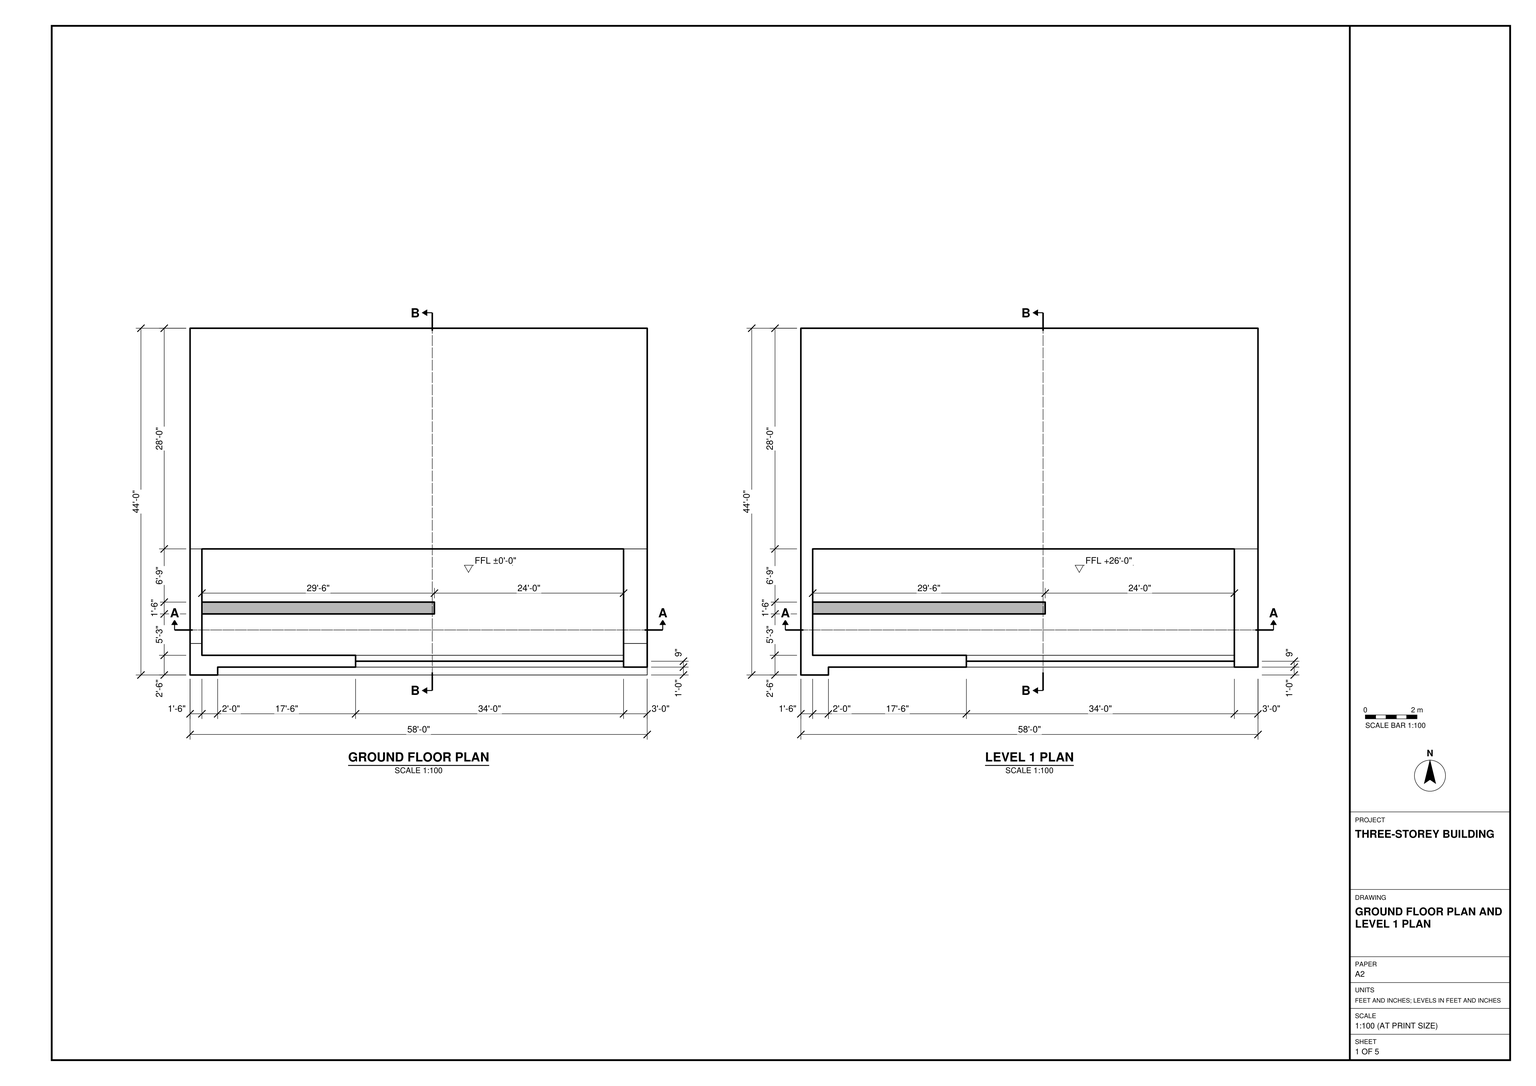
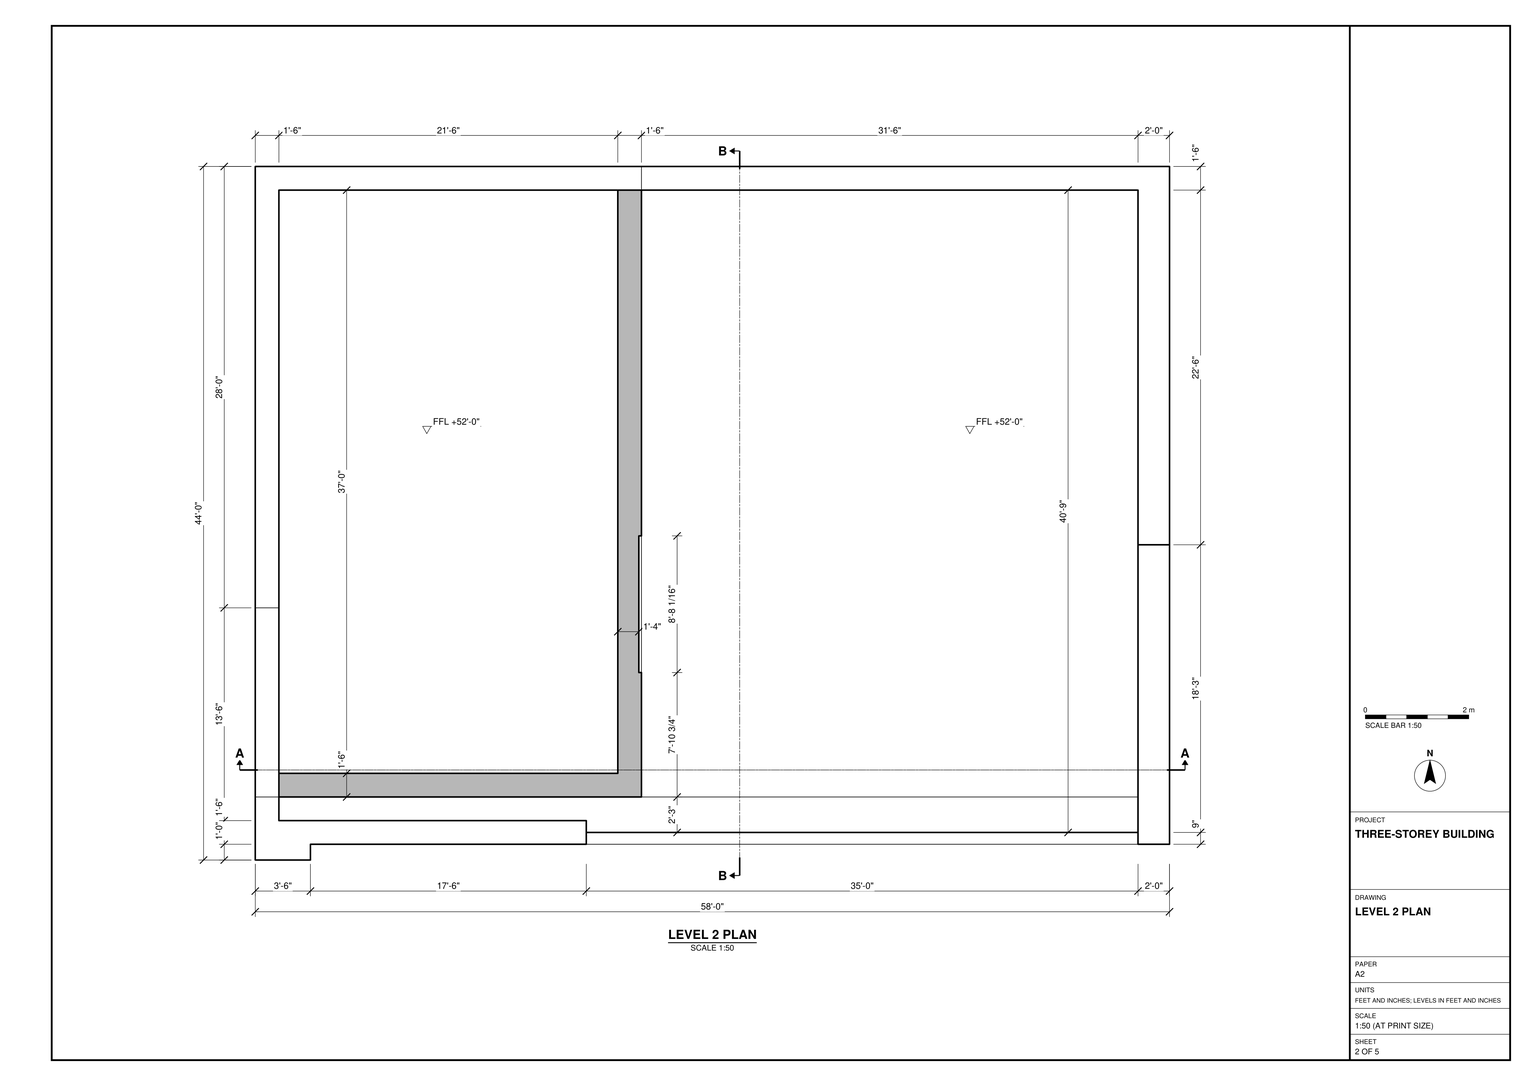
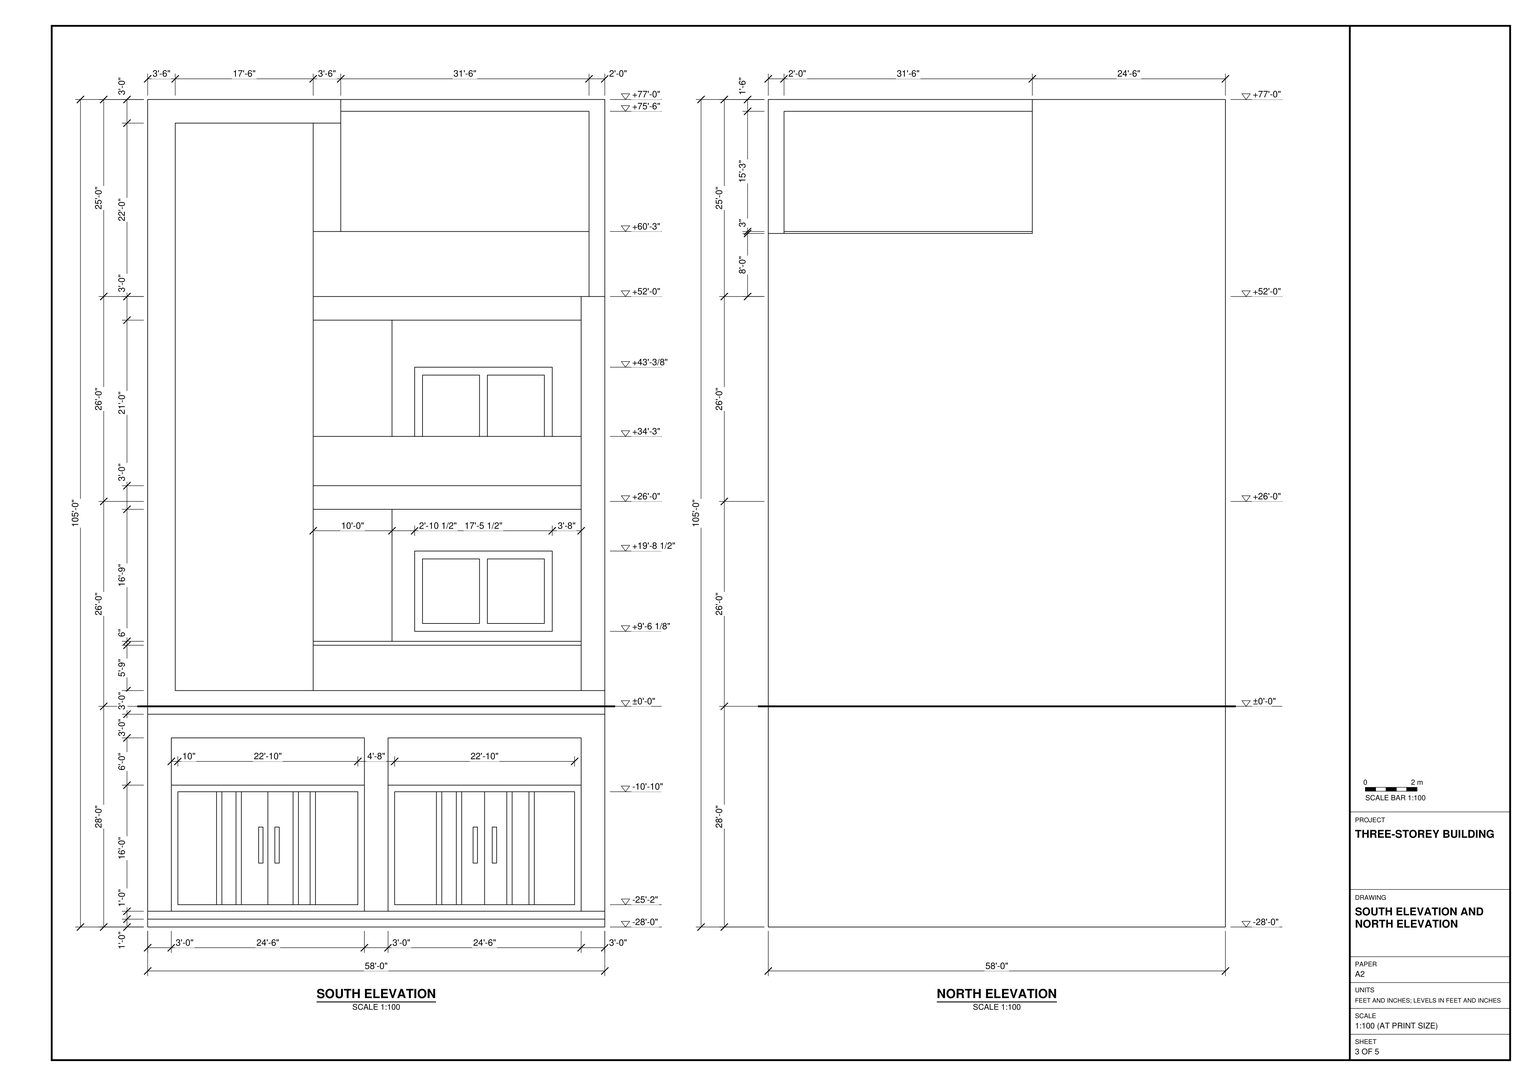
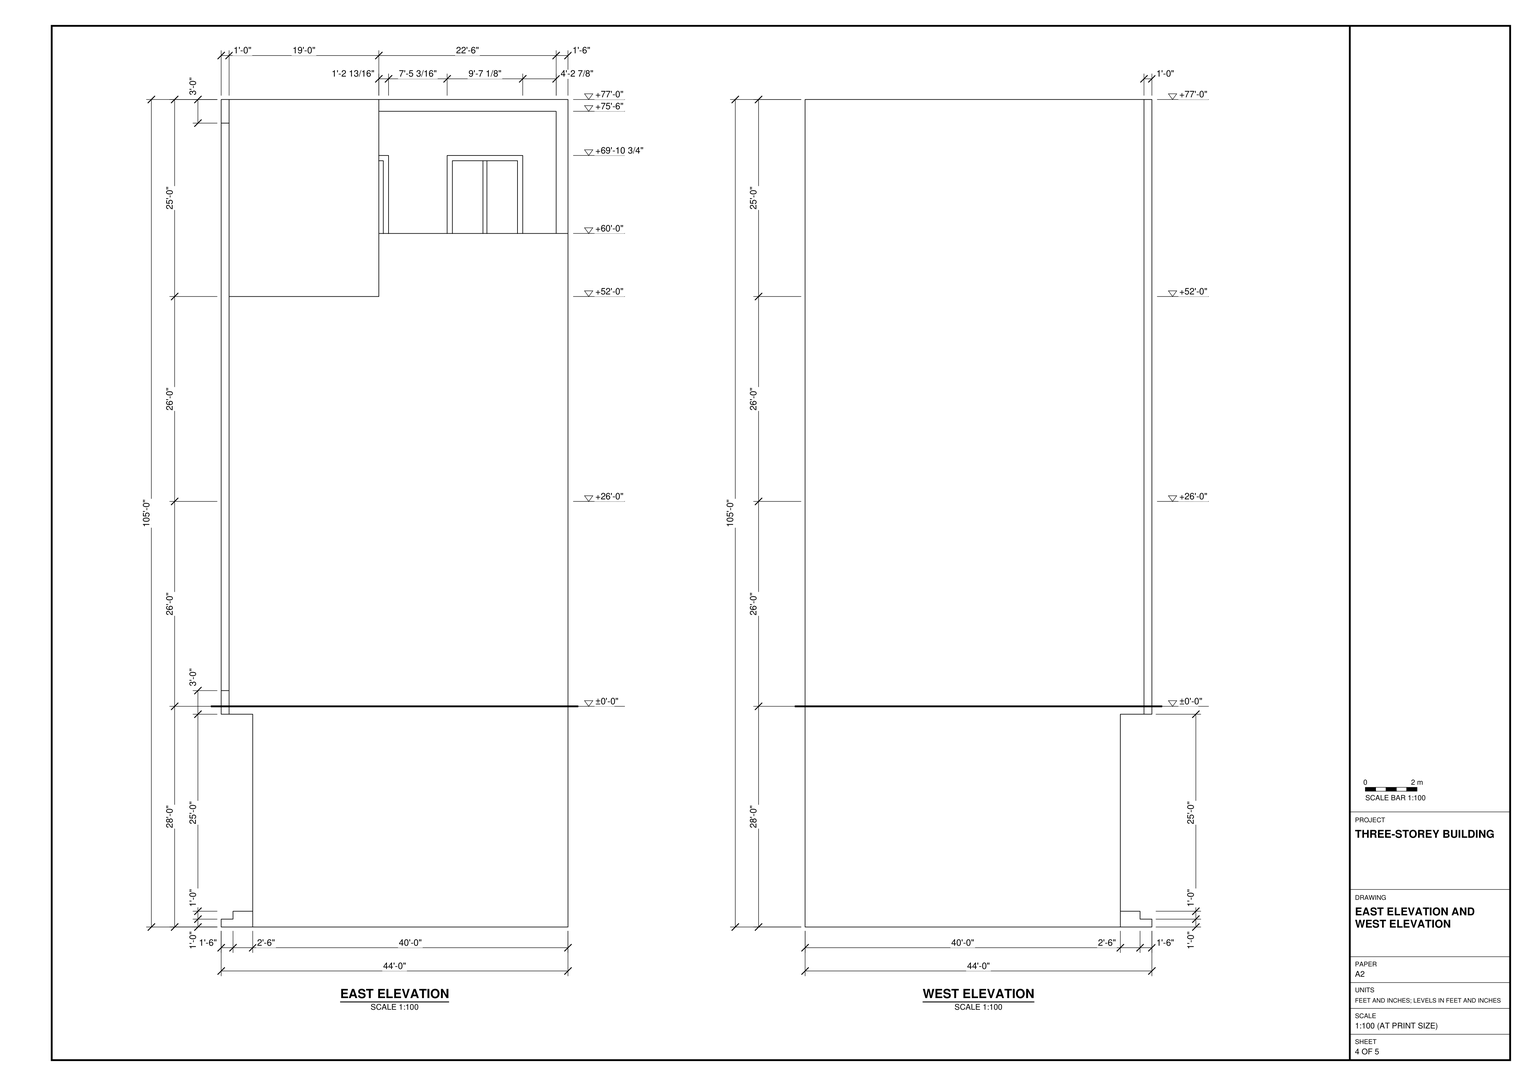
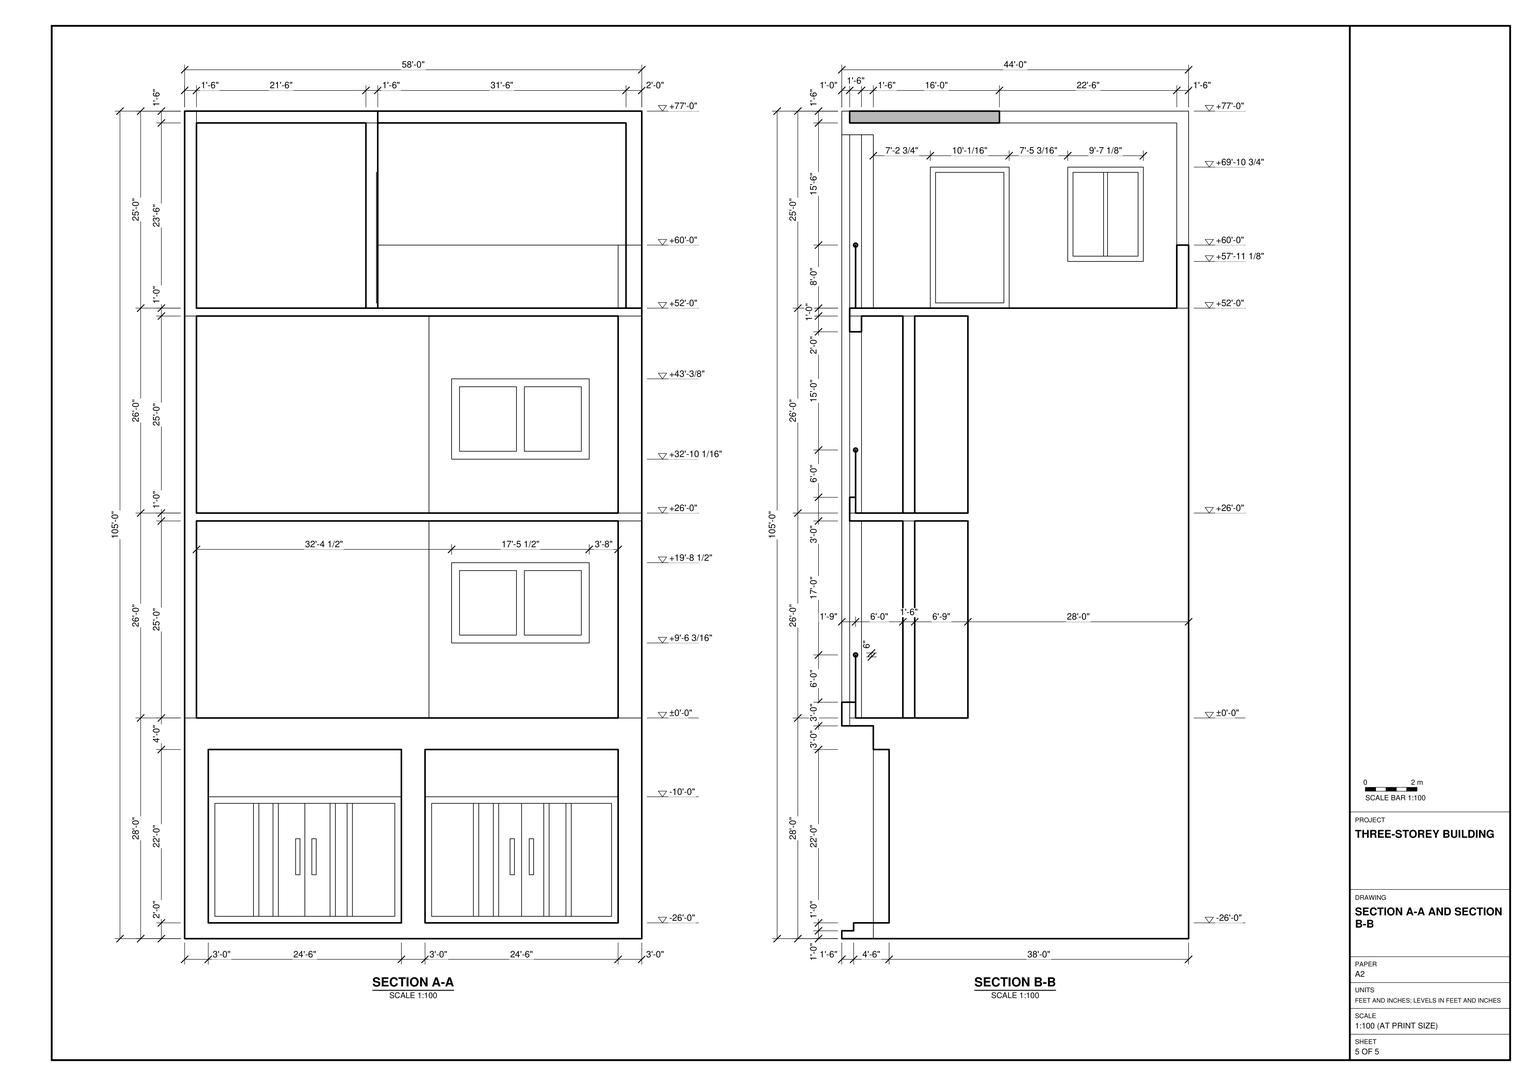
Build the three-storey building in SketchUp from task_files/diagram_01.pdf. Work in feet and inches. Set the overall width to 58'-0", depth to 44'-0" and height to 105'-0". Use ±0'-0" for the ground floor, +26'-0" for level 1 and +52'-0" for level 2. The ground floor is not the bottom of the model: the entrance bays lie below it, with the base at -28'-0" and the top of the building at +77'-0".

Use the plans to lay out the perimeter walls, floor slabs and stepped south edge. Match the wall thicknesses as drawn. Repeat the south-side layout on the ground floor and level 1. On level 2, form the narrower west bay with its L-shaped wall. Use the elevations to model the two framed entrance bays, the tall uninterrupted field on the left of the south facade and the stacked window units to its right. Follow the sheets for the roof outline and the large upper opening on the north side.

Keep walls, slabs and roof elements in separate groups or components. Group each furniture or joinery piece shown separately, and use components for repeated parts. Any decor or loose items shown may be suitable library components. Save one SketchUp model as output_files/three_storey_building_with_paired_south_entrance_bays.skp.

# SketchUp Ruby script. Lengths in inches.
U = 1.inch
M = Sketchup.active_model
def pt(a) = Geom::Point3d.new(a.map { |v| v * U })
def face(e, loops, mat)
  f = e.add_face(loops[0].map { |a| pt(a) })
  loops[1..].each { |l| e.add_face(l.map { |a| pt(a) }).erase! }
  f.material = f.back_material = mat if mat
  f
end
# faces: each face lists its corners as indices into pts; further lists are holes
def faces(e, pts, list, mat = nil) = list.each { |f| face(e, (f[0].is_a?(Array) ? f : [f]).map { |l| l.map { |i| pts[i] } }, mat) }
# xy, xz, yz: faces in a plane at the given z, y or x. An outline is a flat list of corners, or four numbers for a rectangle; further outlines are holes
def ring(l) = l.size == 4 ? [[l[0], l[1]], [l[2], l[1]], [l[2], l[3]], [l[0], l[3]]] : l.each_slice(2).to_a
def flat(e, list, mat, &to3) = list.each { |f| face(e, (f[0].is_a?(Array) ? f : [f]).map { |l| ring(l).map { |u, v| to3.(u, v) } }, mat) }
def xy(e, z, list, mat = nil) = flat(e, list, mat) { |x, y| [x, y, z] }
def xz(e, y, list, mat = nil) = flat(e, list, mat) { |x, z| [x, y, z] }
def yz(e, x, list, mat = nil) = flat(e, list, mat) { |y, z| [x, y, z] }
def lines(e, pts, list) = list.each { |a, b| e.add_line(pt(pts[a]), pt(pts[b])) }
# prism: a flat outline (further loops are holes) pulled along v
def prism(e, loops, v, mat = nil)
  f = face(e, loops, mat); d = Geom::Vector3d.new(v.map { |x| x * U })
  f.pushpull(f.normal.samedirection?(d) ? d.length : -d.length)
end
def box(e, o, s, mat = nil) = prism(e, [[o, [o[0] + s[0], o[1], o[2]], [o[0] + s[0], o[1] + s[1], o[2]], [o[0], o[1] + s[1], o[2]]]], [0, 0, s[2]], mat)
def at(x, y, z, deg = 0) = Geom::Transformation.translation(pt([x, y, z])) * Geom::Transformation.rotation(ORIGIN, Z_AXIS, deg.degrees)
def axes(o, x, y, z) = Geom::Transformation.new([*x, 0, *y, 0, *z, 0, *pt(o).to_a, 1])
def part(name) = M.definitions.add(name)
# library, detail: a bought-in or finely detailed component or shape, given as its bounding box
def library(name, o, s) = part(name).tap { |d| box(d.entities, o, s) }
def detail(e, o, s) = box(e.add_group.entities, o, s)
def put(e, d, t, mat = nil) = e.add_instance(d, t).tap { |i| i.material = mat if mat }
def group(e, t, mat = nil) = e.add_group.tap { |g| g.transformation = t; g.material = mat if mat }.entities
root = M.entities
M.materials.add("[0021_DarkRed]").color = [76, 0, 0]
M.materials.add("[0037_SandyBrown]").color = [104, 70, 41]
M.materials.add("[0039_DarkOrange]").color = [198, 109, 0]
M.materials.add("[0118_Thistle]").color = [216, 191, 216]
M.materials.add("[0119_RosyBrown]").color = [96, 73, 73]
M.materials.add("[0132_LightGray]").color = [169, 169, 169]
M.materials.add("[0136_Charcoal]").color = [35, 35, 35]
M.materials.add("[Checker Plate]").color = [145, 145, 145]
M.materials.add("[Grass Dark Green]").color = [106, 157, 55]
M.materials.add("[Sandstone]").color = [118, 81, 52]
M.materials.add("[Stone Masonry Multi]").color = [165, 159, 149]
M.materials.add("[Tile Veriegated Stone]").color = [171, 137, 112]
M.materials.add("[Translucent Glass Blue]").color = [59, 88, 140]
M.materials["[Translucent Glass Blue]"].alpha = 0.5
M.materials.add("[Translucent Glass Blue]1").color = [75, 112, 178]
M.materials["[Translucent Glass Blue]1"].alpha = 0.5
M.materials.add("[Translucent Glass Gray]").color = [128, 128, 128]
M.materials["[Translucent Glass Gray]"].alpha = 0.5
M.materials.add("[Wood Bamboo]").color = [177, 105, 43]
xy(root,-12,[[0,0,696,528]])
xy(root,0,[[0,0,696,18]],"[Sandstone]")
xy(root,12,[[0,18,696,18,696,48,660,48,660,72,366,72,366,48,330,48,330,72,36,72,36,48,0,48]],"[Sandstone]")
xy(root,85.31,[[168.9375,71,175.625,72],[193.625,71,200.3125,72],[495.4375,71,502.125,72],[524.625,71,531.3125,72]])
xy(root,140.18,[[168.9375,71,175.625,72],[193.625,71,200.3125,72],[495.4375,71,502.125,72],[524.625,71,531.3125,72]])
xy(root,276,[[36,48,330,72],[366,48,660,72]],"[0119_RosyBrown]")
xy(root,312,[[0,0,696,48]],"[Wood Bamboo]")
xy(root,324,[[252,21,660,30],[18,93,372,111]])
xy(root,324,[[18,30,660,30,660,192,18,192,18,111,372,111,372,93,18,93]],"[Grass Dark Green]")
xy(root,348,[[252,12,660,21]])
xy(root,348,[[42,0,696,12]],"[Wood Bamboo]")
xy(root,624,[[252,12,252,30,18,30,18,93,372,93,372,111,18,111,18,192,660,192,660,12]],"[0118_Thistle]")
xy(root,636,[[252,21,660,30],[18,93,372,111]])
xy(root,636,[[18,30,660,30,660,192,18,192,18,111,372,111,372,93,18,93]],"[Grass Dark Green]")
xy(root,660,[[252,12,660,21]])
xy(root,912,[[252,12,660,30]],"[0118_Thistle]")
xy(root,936,[[18,30,18,93,372,93,372,111,18,111,18,192,660,192,660,30]],"[0118_Thistle]")
xy(root,948,[[252,12,672,21],[672,12,696,240],[252,21,672,21,672,48,18,48,18,30,252,30],[294,48,672,510],[18,66,276,510],
  [276,66,294,510]])
xy(root,956,[[292,142.73,294,246.79]])
xy(root,1027.125,[[293,352,294,398.5625],[293,404.5625,294,451.125]])
xy(root,1044,[[672,240,696,240,696,528,294,528,294,510,672,510]])
xy(root,1154.75,[[292,142.73,294,246.79],[293,352,294,398.5625],[293,404.5625,294,451.125]])
xy(root,1212,[[42,0,42,12,252,12,252,30,18,30,18,48,294,48,294,0]],"[Wood Bamboo]")
xy(root,1230,[[294,12,672,240],[18,48,294,66],[18,66,276,510]])
xy(root,1248,[[0,12,294,528],[294,12,696,240]])
xy(root,1248,[[0,0,294,12]],"[Wood Bamboo]")
xz(root,0,[[0,-12,696,0]],"[Sandstone]")
xz(root,0,[[0,312,696,312,696,348,42,348,42,1212,294,1212,294,1248,0,1248]],"[Wood Bamboo]")
xz(root,12,[[660,348,696,948],[672,948,696,948,696,1248,294,1248,294,1230,672,1230]])
xz(root,12,[[42,348,252,1212]],"[Checker Plate]")
xz(root,12,[[252,624,660,660],[252,912,660,948]],"[Wood Bamboo]")
xz(root,18,[[0,0,696,12]],"[Sandstone]")
xz(root,21,[[252,324,660,348],[252,417,660,420],[252,636,660,660],[252,729,660,732],[252,1041,672,1044]])
xz(root,21,[[252,348,660,416],[252,416,660,417],[252,660,660,729],[252,948,672,1041]],"[Translucent Glass Gray]")
xz(root,30,[[18,636,252,936],[252,912,660,936],[18,948,252,1212]])
xz(root,30,[[18,324,252,624]],"[Tile Veriegated Stone]")
xz(root,48,[[0,12,36,12,36,276,330,276,330,12,366,12,366,276,660,276,660,12,696,12,696,312,0,312]],"[0119_RosyBrown]")
xz(root,48,[[18,948,294,1212]],"[Stone Masonry Multi]")
xz(root,66,[[18,948,276,1230]])
xz(root,71,[[168.9375,85.31,175.625,140.18],[193.625,85.31,200.3125,140.18],[495.4375,85.31,502.125,140.18],[524.625,85.31,531.3125,140.18]])
xz(root,72,[[[36,12,330,204],[46,22,320,194]],[[366,12,660,204],[376,22,650,194]],[46,22,104.84,194],[112.98,22,134.52,194],[[142.67,22,183,194],[168.9375,85.31,175.625,140.18]],
  [[183,22,221.4,194],[193.625,85.31,200.3125,140.18]],[229.54,22,247.34,194],[255.48,22,320,194],[376,22,439.65,194],[447.79,22,469.96,194],
  [[478.11,22,513,194],[495.4375,85.31,502.125,140.18]],[[513,22,546.77,194],[524.625,85.31,531.3125,140.18]],[554.92,22,580.52,194],[588.67,22,650,194]],"[0037_SandyBrown]")
xz(root,72,[[104.84,22,112.98,194],[134.52,22,142.67,194],[221.4,22,229.54,194],[247.34,22,255.48,194],[439.65,22,447.79,194],
  [469.96,22,478.11,194],[546.77,22,554.92,194],[580.52,22,588.67,194]],"[0039_DarkOrange]")
xz(root,72,[[36,204,330,276],[366,204,660,276]],"[0136_Charcoal]")
xz(root,93,[[18,324,372,624],[18,636,372,936]],"[Tile Veriegated Stone]")
xz(root,111,[[18,636,372,936]])
xz(root,111,[[18,324,372,624]],"[Tile Veriegated Stone]")
xz(root,142.73,[[292,956,294,1154.75]])
xz(root,192,[[[406.48,438.16,615.98,560.47],[517.23,450.16,603.98,548.47],[418.48,450.16,505.23,548.47]],[[406.48,718.03,615.98,840.34],[418.48,730.03,505.23,828.34],[517.23,730.03,603.98,828.34]]],"[0021_DarkRed]")
xz(root,192,[[[18,324,660,624],[406.48,438.16,615.98,560.47]],[[18,636,660,936],[406.48,718.03,615.98,840.34]]],"[Tile Veriegated Stone]")
xz(root,192,[[418.48,450.16,505.23,548.47],[517.23,450.16,603.98,548.47],[418.48,730.03,505.23,828.34],[517.23,730.03,603.98,828.34]],"[Translucent Glass Blue]")
xz(root,240,[[672,948,696,1044],[672,1044,672,1230,294,1230,294,1248,696,1248,696,1044]])
xz(root,246.79,[[292,956,294,1154.75]])
xz(root,352,[[293,1027.125,294,1154.75]])
xz(root,398.5625,[[293,1027.125,294,1154.75]])
xz(root,404.5625,[[293,1027.125,294,1154.75]])
xz(root,451.125,[[293,1027.125,294,1154.75]])
xz(root,510,[[18,948,276,1230],[276,948,294,1230],[294,948,660,1044],[660,948,672,1044]])
xz(root,528,[[0,-12,0,1248,294,1248,294,1044,696,1044,696,-12]])
yz(root,0,[[0,-12,0,0,18,0,18,12,48,12,48,-12],[48,-12,48,312,12,312,12,1248,528,1248,528,-12]])
yz(root,0,[[0,312,12,1248]],"[Wood Bamboo]")
yz(root,18,[[93,324,111,624],[93,636,111,936],[30,948,48,1212],[48,948,66,1230],[66,948,510,1230]])
yz(root,18,[[30,324,93,624],[111,324,192,624],[30,636,93,936],[111,636,192,936]],"[Tile Veriegated Stone]")
yz(root,36,[[48,12,72,276]],"[0119_RosyBrown]")
yz(root,42,[[0,348,12,1212]],"[Wood Bamboo]")
yz(root,168.9375,[[71,85.31,72,140.18]])
yz(root,175.625,[[71,85.31,72,140.18]])
yz(root,193.625,[[71,85.31,72,140.18]])
yz(root,200.3125,[[71,85.31,72,140.18]])
yz(root,252,[[21,417,20.6875,417.02,20.375,417.07,20.07,417.15,19.78,417.26,19.5,417.4,19.24,417.57,18.99,417.77,18.77,417.99,18.57,418.24,18.4,418.5,18.26,418.78,18.15,419.07,18.07,419.375,18.02,419.6875,18,420,18.02,420.3125,18.07,420.625,18.15,420.93,18.26,421.22,18.4,421.5,18.57,421.76,18.77,422.01,18.99,422.23,19.24,422.43,19.5,422.6,19.78,422.74,20.07,422.85,20.375,422.93,20.6875,422.98,21,423,21.3125,422.98,21.625,422.93,21.93,422.85,22.22,422.74,22.5,422.6,22.76,422.43,23.01,422.23,23.23,422.01,23.43,421.76,23.6,421.5,23.74,421.22,23.85,420.93,23.93,420.625,23.98,420.3125,24,420,23.98,419.6875,23.93,419.375,23.85,419.07,23.74,418.78,23.6,418.5,23.43,418.24,23.23,417.99,23.01,417.77,22.76,417.57,22.5,417.4,22.22,417.26,21.93,417.15,21.625,417.07,21.3125,417.02],[12,636,21,660],[12,912,30,936]])
yz(root,252,[[[12,948,30,1212],[21,1041,20.6875,1041.02,20.375,1041.07,20.07,1041.15,19.78,1041.26,19.5,1041.4,19.24,1041.57,18.99,1041.77,18.77,1041.99,18.57,1042.24,18.4,1042.5,18.26,1042.78,18.15,1043.07,18.07,1043.375,18.02,1043.6875,18,1044,18.02,1044.3125,18.07,1044.625,18.15,1044.93,18.26,1045.22,18.4,1045.5,18.57,1045.76,18.77,1046.01,18.99,1046.23,19.24,1046.43,19.5,1046.6,19.78,1046.74,20.07,1046.85,20.375,1046.93,20.6875,1046.98,21,1047,21.3125,1046.98,21.625,1046.93,21.93,1046.85,22.22,1046.74,22.5,1046.6,22.76,1046.43,23.01,1046.23,23.23,1046.01,23.43,1045.76,23.6,1045.5,23.74,1045.22,23.85,1044.93,23.93,1044.625,23.98,1044.3125,24,1044,23.98,1043.6875,23.93,1043.375,23.85,1043.07,23.74,1042.78,23.6,1042.5,23.43,1042.24,23.23,1041.99,23.01,1041.77,22.76,1041.57,22.5,1041.4,22.22,1041.26,21.93,1041.15,21.625,1041.07,21.3125,1041.02]]],"[0132_LightGray]")
yz(root,252,[[21,324,30,324,30,624,12,624,12,348,21,348],[[21,636,30,636,30,912,12,912,12,660,21,660],[21,729,20.22,729.1,19.5,729.4,18.88,729.88,18.4,730.5,18.1,731.22,18,732,18.1,732.78,18.4,733.5,18.88,734.12,19.5,734.6,20.22,734.9,21,735,21.78,734.9,22.5,734.6,23.12,734.12,23.6,733.5,23.9,732.78,24,732,23.9,731.22,23.6,730.5,23.12,729.88,22.5,729.4,21.78,729.1]]],"[Tile Veriegated Stone]")
yz(root,276,[[66,948,510,1230]])
yz(root,292,[[142.73,956,246.79,1154.75]],"[Translucent Glass Blue]1")
yz(root,293,[[352,1027.125,398.5625,1154.75],[404.5625,1027.125,451.125,1154.75]],"[Translucent Glass Blue]1")
yz(root,294,[[12,1230,240,1248]])
yz(root,294,[[510,1044,528,1044,528,1248,240,1248,240,1230,510,1230]],"[0132_LightGray]")
yz(root,294,[[[134.73,948,254.79,1162.75],[142.73,956,246.79,1154.75]],[[344,1019.125,459.125,1162.75],[352,1027.125,451.125,1154.75]],[398.5625,1027.125,404.5625,1154.75]],"[0136_Charcoal]")
yz(root,294,[[[48,948,134.73,948,134.73,1162.75,254.79,1162.75,254.79,948,510,948,510,1230,12,1230,12,1248,0,1248,0,1212,48,1212],[344,1019.125,459.125,1162.75]]],"[Stone Masonry Multi]")
yz(root,330,[[48,12,72,276]],"[0119_RosyBrown]")
yz(root,366,[[48,12,72,276]],"[0119_RosyBrown]")
yz(root,372,[[93,324,111,624],[93,636,111,936]],"[Tile Veriegated Stone]")
yz(root,495.4375,[[71,85.31,72,140.18]])
yz(root,502.125,[[71,85.31,72,140.18]])
yz(root,524.625,[[71,85.31,72,140.18]])
yz(root,531.3125,[[71,85.31,72,140.18]])
yz(root,660,[[21,417,21.3125,417.02,21.625,417.07,21.93,417.15,22.22,417.26,22.5,417.4,22.76,417.57,23.01,417.77,23.23,417.99,23.43,418.24,23.6,418.5,23.74,418.78,23.85,419.07,23.93,419.375,23.98,419.6875,24,420,23.98,420.3125,23.93,420.625,23.85,420.93,23.74,421.22,23.6,421.5,23.43,421.76,23.23,422.01,23.01,422.23,22.76,422.43,22.5,422.6,22.22,422.74,21.93,422.85,21.625,422.93,21.3125,422.98,21,423,20.6875,422.98,20.375,422.93,20.07,422.85,19.78,422.74,19.5,422.6,19.24,422.43,18.99,422.23,18.77,422.01,18.57,421.76,18.4,421.5,18.26,421.22,18.15,420.93,18.07,420.625,18.02,420.3125,18,420,18.02,419.6875,18.07,419.375,18.15,419.07,18.26,418.78,18.4,418.5,18.57,418.24,18.77,417.99,18.99,417.77,19.24,417.57,19.5,417.4,19.78,417.26,20.07,417.15,20.375,417.07,20.6875,417.02],[12,636,21,660],[21,729,21.78,729.1,22.5,729.4,23.12,729.88,23.6,730.5,23.9,731.22,24,732,23.9,732.78,23.6,733.5,23.12,734.12,22.5,734.6,21.78,734.9,21,735,20.22,734.9,19.5,734.6,18.88,734.12,18.4,733.5,18.1,732.78,18,732,18.1,731.22,18.4,730.5,18.88,729.88,19.5,729.4,20.22,729.1],[12,912,30,936]])
yz(root,660,[[48,12,72,276]],"[0119_RosyBrown]")
yz(root,660,[[[21,324,21,348,12,348,12,624,192,624,192,324],[21,417,21.3125,417.02,21.625,417.07,21.93,417.15,22.22,417.26,22.5,417.4,22.76,417.57,23.01,417.77,23.23,417.99,23.43,418.24,23.6,418.5,23.74,418.78,23.85,419.07,23.93,419.375,23.98,419.6875,24,420,23.98,420.3125,23.93,420.625,23.85,420.93,23.74,421.22,23.6,421.5,23.43,421.76,23.23,422.01,23.01,422.23,22.76,422.43,22.5,422.6,22.22,422.74,21.93,422.85,21.625,422.93,21.3125,422.98,21,423,20.6875,422.98,20.375,422.93,20.07,422.85,19.78,422.74,19.5,422.6,19.24,422.43,18.99,422.23,18.77,422.01,18.57,421.76,18.4,421.5,18.26,421.22,18.15,420.93,18.07,420.625,18.02,420.3125,18,420,18.02,419.6875,18.07,419.375,18.15,419.07,18.26,418.78,18.4,418.5,18.57,418.24,18.77,417.99,18.99,417.77,19.24,417.57,19.5,417.4,19.78,417.26,20.07,417.15,20.375,417.07,20.6875,417.02]],[[21,636,21,660,12,660,12,912,30,912,30,936,192,936,192,636],[21,729,21.78,729.1,22.5,729.4,23.12,729.88,23.6,730.5,23.9,731.22,24,732,23.9,732.78,23.6,733.5,23.12,734.12,22.5,734.6,21.78,734.9,21,735,20.22,734.9,19.5,734.6,18.88,734.12,18.4,733.5,18.1,732.78,18,732,18.1,731.22,18.4,730.5,18.88,729.88,19.5,729.4,20.22,729.1]]],"[Tile Veriegated Stone]")
yz(root,672,[[[12,948,240,1230],[21,1041,21.3125,1041.02,21.625,1041.07,21.93,1041.15,22.22,1041.26,22.5,1041.4,22.76,1041.57,23.01,1041.77,23.23,1041.99,23.43,1042.24,23.6,1042.5,23.74,1042.78,23.85,1043.07,23.93,1043.375,23.98,1043.6875,24,1044,23.98,1044.3125,23.93,1044.625,23.85,1044.93,23.74,1045.22,23.6,1045.5,23.43,1045.76,23.23,1046.01,23.01,1046.23,22.76,1046.43,22.5,1046.6,22.22,1046.74,21.93,1046.85,21.625,1046.93,21.3125,1046.98,21,1047,20.6875,1046.98,20.375,1046.93,20.07,1046.85,19.78,1046.74,19.5,1046.6,19.24,1046.43,18.99,1046.23,18.77,1046.01,18.57,1045.76,18.4,1045.5,18.26,1045.22,18.15,1044.93,18.07,1044.625,18.02,1044.3125,18,1044,18.02,1043.6875,18.07,1043.375,18.15,1043.07,18.26,1042.78,18.4,1042.5,18.57,1042.24,18.77,1041.99,18.99,1041.77,19.24,1041.57,19.5,1041.4,19.78,1041.26,20.07,1041.15,20.375,1041.07,20.6875,1041.02]],[240,948,510,1044],[21,1041,21.3125,1041.02,21.625,1041.07,21.93,1041.15,22.22,1041.26,22.5,1041.4,22.76,1041.57,23.01,1041.77,23.23,1041.99,23.43,1042.24,23.6,1042.5,23.74,1042.78,23.85,1043.07,23.93,1043.375,23.98,1043.6875,24,1044,23.98,1044.3125,23.93,1044.625,23.85,1044.93,23.74,1045.22,23.6,1045.5,23.43,1045.76,23.23,1046.01,23.01,1046.23,22.76,1046.43,22.5,1046.6,22.22,1046.74,21.93,1046.85,21.625,1046.93,21.3125,1046.98,21,1047,20.6875,1046.98,20.375,1046.93,20.07,1046.85,19.78,1046.74,19.5,1046.6,19.24,1046.43,18.99,1046.23,18.77,1046.01,18.57,1045.76,18.4,1045.5,18.26,1045.22,18.15,1044.93,18.07,1044.625,18.02,1044.3125,18,1044,18.02,1043.6875,18.07,1043.375,18.15,1043.07,18.26,1042.78,18.4,1042.5,18.57,1042.24,18.77,1041.99,18.99,1041.77,19.24,1041.57,19.5,1041.4,19.78,1041.26,20.07,1041.15,20.375,1041.07,20.6875,1041.02]])
yz(root,696,[[0,-12,48,-12,48,12,18,12,18,0,0,0],[48,-12,528,-12,528,1044,240,1044,240,948,12,948,12,312,48,312],[12,948,240,1248]])
yz(root,696,[[0,312,12,348]],"[Wood Bamboo]")
p = [[660,20.6875,417.02],[660,20.375,417.07],[252,20.375,417.07],[252,20.6875,417.02],[660,21,417],[252,21,417],
  [660,21.3125,417.02],[252,21.3125,417.02],[660,21.625,417.07],[252,21.625,417.07],[660,20.07,417.15],[660,19.78,417.26],
  [252,19.78,417.26],[252,20.07,417.15],[660,21.93,417.15],[252,21.93,417.15],[660,22.22,417.26],[252,22.22,417.26],
  [660,19.5,417.4],[252,19.5,417.4],[660,22.5,417.4],[252,22.5,417.4],[660,19.24,417.57],[252,19.24,417.57],
  [660,22.76,417.57],[252,22.76,417.57],[660,18.99,417.77],[252,18.99,417.77],[660,23.01,417.77],[252,23.01,417.77],
  [660,18.77,417.99],[252,18.77,417.99],[660,23.23,417.99],[252,23.23,417.99],[660,18.57,418.24],[252,18.57,418.24],
  [660,23.43,418.24],[252,23.43,418.24],[660,18.4,418.5],[252,18.4,418.5],[660,23.6,418.5],[252,23.6,418.5],
  [660,18.26,418.78],[252,18.26,418.78],[660,23.74,418.78],[252,23.74,418.78],[660,18.15,419.07],[252,18.15,419.07],
  [660,23.85,419.07],[252,23.85,419.07],[660,18.07,419.375],[252,18.07,419.375],[660,23.93,419.375],[252,23.93,419.375],
  [660,18.02,419.6875],[252,18.02,419.6875],[660,23.98,419.6875],[252,23.98,419.6875],[660,18,420],[252,18,420],
  [660,24,420],[252,24,420],[660,18.02,420.3125],[252,18.02,420.3125],[660,23.98,420.3125],[252,23.98,420.3125],
  [660,18.07,420.625],[252,18.07,420.625],[660,23.93,420.625],[252,23.93,420.625],[660,18.15,420.93],[252,18.15,420.93],
  [660,23.85,420.93],[252,23.85,420.93],[660,18.26,421.22],[252,18.26,421.22],[660,23.74,421.22],[252,23.74,421.22],
  [660,18.4,421.5],[252,18.4,421.5],[660,23.6,421.5],[252,23.6,421.5],[660,18.57,421.76],[252,18.57,421.76],
  [660,23.43,421.76],[252,23.43,421.76],[660,18.77,422.01],[252,18.77,422.01],[660,23.23,422.01],[252,23.23,422.01],
  [660,18.99,422.23],[252,18.99,422.23],[660,23.01,422.23],[252,23.01,422.23],[660,19.24,422.43],[252,19.24,422.43],
  [660,22.76,422.43],[252,22.76,422.43],[660,19.5,422.6],[252,19.5,422.6],[660,22.5,422.6],[252,22.5,422.6],
  [660,19.78,422.74],[252,19.78,422.74],[660,22.22,422.74],[252,22.22,422.74],[660,20.07,422.85],[252,20.07,422.85],
  [660,21.93,422.85],[252,21.93,422.85],[660,20.375,422.93],[252,20.375,422.93],[660,20.6875,422.98],[252,20.6875,422.98],
  [660,21.3125,422.98],[660,21.625,422.93],[252,21.625,422.93],[252,21.3125,422.98],[660,21,423],[252,21,423],
  [660,21,729],[660,20.22,729.1],[252,20.22,729.1],[252,21,729],[660,21.78,729.1],[252,21.78,729.1],
  [660,19.5,729.4],[252,19.5,729.4],[660,22.5,729.4],[252,22.5,729.4],[660,18.88,729.88],[252,18.88,729.88],
  [660,23.12,729.88],[252,23.12,729.88],[660,18.4,730.5],[252,18.4,730.5],[660,23.6,730.5],[252,23.6,730.5],
  [660,18.1,731.22],[252,18.1,731.22],[660,23.9,731.22],[252,23.9,731.22],[660,18,732],[252,18,732],
  [660,24,732],[252,24,732],[660,18.1,732.78],[252,18.1,732.78],[660,23.9,732.78],[252,23.9,732.78],
  [660,18.4,733.5],[252,18.4,733.5],[660,23.6,733.5],[252,23.6,733.5],[660,18.88,734.12],[252,18.88,734.12],
  [660,23.12,734.12],[252,23.12,734.12],[660,19.5,734.6],[252,19.5,734.6],[660,22.5,734.6],[252,22.5,734.6],
  [660,20.22,734.9],[252,20.22,734.9],[660,21.78,734.9],[252,21.78,734.9],[660,21,735],[252,21,735],
  [672,20.6875,1041.02],[672,20.375,1041.07],[252,20.375,1041.07],[252,20.6875,1041.02],[672,21,1041],[252,21,1041],
  [672,21.3125,1041.02],[252,21.3125,1041.02],[672,21.625,1041.07],[252,21.625,1041.07],[672,20.07,1041.15],[672,19.78,1041.26],
  [252,19.78,1041.26],[252,20.07,1041.15],[672,21.93,1041.15],[252,21.93,1041.15],[672,22.22,1041.26],[252,22.22,1041.26],
  [672,19.5,1041.4],[252,19.5,1041.4],[672,22.5,1041.4],[252,22.5,1041.4],[672,19.24,1041.57],[252,19.24,1041.57],
  [672,22.76,1041.57],[252,22.76,1041.57],[672,18.99,1041.77],[252,18.99,1041.77],[672,23.01,1041.77],[252,23.01,1041.77],
  [672,18.77,1041.99],[252,18.77,1041.99],[672,23.23,1041.99],[252,23.23,1041.99],[672,18.57,1042.24],[252,18.57,1042.24],
  [672,23.43,1042.24],[252,23.43,1042.24],[672,18.4,1042.5],[252,18.4,1042.5],[672,23.6,1042.5],[252,23.6,1042.5],
  [672,18.26,1042.78],[252,18.26,1042.78],[672,23.74,1042.78],[252,23.74,1042.78],[672,18.15,1043.07],[252,18.15,1043.07],
  [672,23.85,1043.07],[252,23.85,1043.07],[672,18.07,1043.375],[252,18.07,1043.375],[672,23.93,1043.375],[252,23.93,1043.375],
  [672,18.02,1043.6875],[252,18.02,1043.6875],[672,23.98,1043.6875],[252,23.98,1043.6875],[672,18,1044],[252,18,1044],
  [672,24,1044],[252,24,1044],[672,18.02,1044.3125],[252,18.02,1044.3125],[672,23.98,1044.3125],[252,23.98,1044.3125],
  [672,18.07,1044.625],[252,18.07,1044.625],[672,23.93,1044.625],[252,23.93,1044.625],[672,18.15,1044.93],[252,18.15,1044.93],
  [672,23.85,1044.93],[252,23.85,1044.93],[672,18.26,1045.22],[252,18.26,1045.22],[672,23.74,1045.22],[252,23.74,1045.22],
  [672,18.4,1045.5],[252,18.4,1045.5],[672,23.6,1045.5],[252,23.6,1045.5],[672,18.57,1045.76],[252,18.57,1045.76],
  [672,23.43,1045.76],[252,23.43,1045.76],[672,18.77,1046.01],[252,18.77,1046.01],[672,23.23,1046.01],[252,23.23,1046.01],
  [672,18.99,1046.23],[252,18.99,1046.23],[672,23.01,1046.23],[252,23.01,1046.23],[672,19.24,1046.43],[252,19.24,1046.43],
  [672,22.76,1046.43],[252,22.76,1046.43],[672,19.5,1046.6],[252,19.5,1046.6],[672,22.5,1046.6],[252,22.5,1046.6],
  [672,19.78,1046.74],[252,19.78,1046.74],[672,22.22,1046.74],[252,22.22,1046.74],[672,20.07,1046.85],[252,20.07,1046.85],
  [672,21.93,1046.85],[252,21.93,1046.85],[672,20.375,1046.93],[252,20.375,1046.93],[672,20.6875,1046.98],[252,20.6875,1046.98],
  [672,21.3125,1046.98],[672,21.625,1046.93],[252,21.625,1046.93],[252,21.3125,1046.98],[672,21,1047],[252,21,1047],
  [696,192,324],[660,192,324],[696,192,624],[660,192,624],[696,192,636],[660,192,636],
  [696,192,936],[660,192,936],[0,48,936],[18,48,936],[18,192,324],[0,192,324],
  [252,12,324],[252,21,324],[18,192,936],[0,192,936],[660,48,936],[696,48,936],
  [660,21,324],[660,12,324],[18,510,1230],[18,510,1248],[294,510,948],[294,528,948]]
faces(root,p,[[0,1,2,3],[4,0,3,5],[6,4,5,7],[8,6,7,9],[10,11,12,13],[1,10,13,2],[14,8,9,15],[16,14,15,17],
  [11,18,19,12],[20,16,17,21],[18,22,23,19],[24,20,21,25],[22,26,27,23],[28,24,25,29],[26,30,31,27],[32,28,29,33],
  [30,34,35,31],[36,32,33,37],[34,38,39,35],[40,36,37,41],[38,42,43,39],[44,40,41,45],[42,46,47,43],[48,44,45,49],
  [46,50,51,47],[52,48,49,53],[50,54,55,51],[56,52,53,57],[54,58,59,55],[60,56,57,61],[58,62,63,59],[64,60,61,65],
  [62,66,67,63],[68,64,65,69],[66,70,71,67],[72,68,69,73],[70,74,75,71],[76,72,73,77],[74,78,79,75],[80,76,77,81],
  [78,82,83,79],[84,80,81,85],[82,86,87,83],[88,84,85,89],[86,90,91,87],[92,88,89,93],[90,94,95,91],[96,92,93,97],
  [94,98,99,95],[100,96,97,101],[98,102,103,99],[104,100,101,105],[102,106,107,103],[108,104,105,109],[106,110,111,107],[110,112,113,111],
  [114,115,116,117],[115,108,109,116],[112,118,119,113],[118,114,117,119],[120,121,122,123],[124,120,123,125],[121,126,127,122],[128,124,125,129],
  [126,130,131,127],[132,128,129,133],[130,134,135,131],[136,132,133,137],[134,138,139,135],[140,136,137,141],[138,142,143,139],[144,140,141,145],
  [142,146,147,143],[148,144,145,149],[146,150,151,147],[152,148,149,153],[150,154,155,151],[156,152,153,157],[154,158,159,155],[160,156,157,161],
  [158,162,163,159],[164,160,161,165],[162,166,167,163],[166,164,165,167],[168,169,170,171],[172,168,171,173],[174,172,173,175],[176,174,175,177],
  [178,179,180,181],[169,178,181,170],[182,176,177,183],[184,182,183,185],[179,186,187,180],[188,184,185,189],[186,190,191,187],[192,188,189,193],
  [190,194,195,191],[196,192,193,197],[194,198,199,195],[200,196,197,201],[198,202,203,199],[204,200,201,205],[202,206,207,203],[208,204,205,209],
  [206,210,211,207],[212,208,209,213],[210,214,215,211],[216,212,213,217],[214,218,219,215],[220,216,217,221],[218,222,223,219],[224,220,221,225],
  [222,226,227,223],[228,224,225,229],[226,230,231,227],[232,228,229,233],[230,234,235,231],[236,232,233,237],[234,238,239,235],[240,236,237,241],
  [238,242,243,239],[244,240,241,245],[242,246,247,243],[248,244,245,249],[246,250,251,247],[252,248,249,253],[250,254,255,251],[256,252,253,257],
  [254,258,259,255],[260,256,257,261],[258,262,263,259],[264,260,261,265],[262,266,267,263],[268,264,265,269],[266,270,271,267],[272,268,269,273],
  [270,274,275,271],[276,272,273,277],[274,278,279,275],[278,280,281,279],[282,283,284,285],[283,276,277,284],[280,286,287,281],[286,282,285,287]])
lines(root,p,[[288,289],[290,291],[292,293],[294,295],[296,297],[298,299],[300,301],[302,303],[304,305],[306,307],[308,309],[310,311]])
